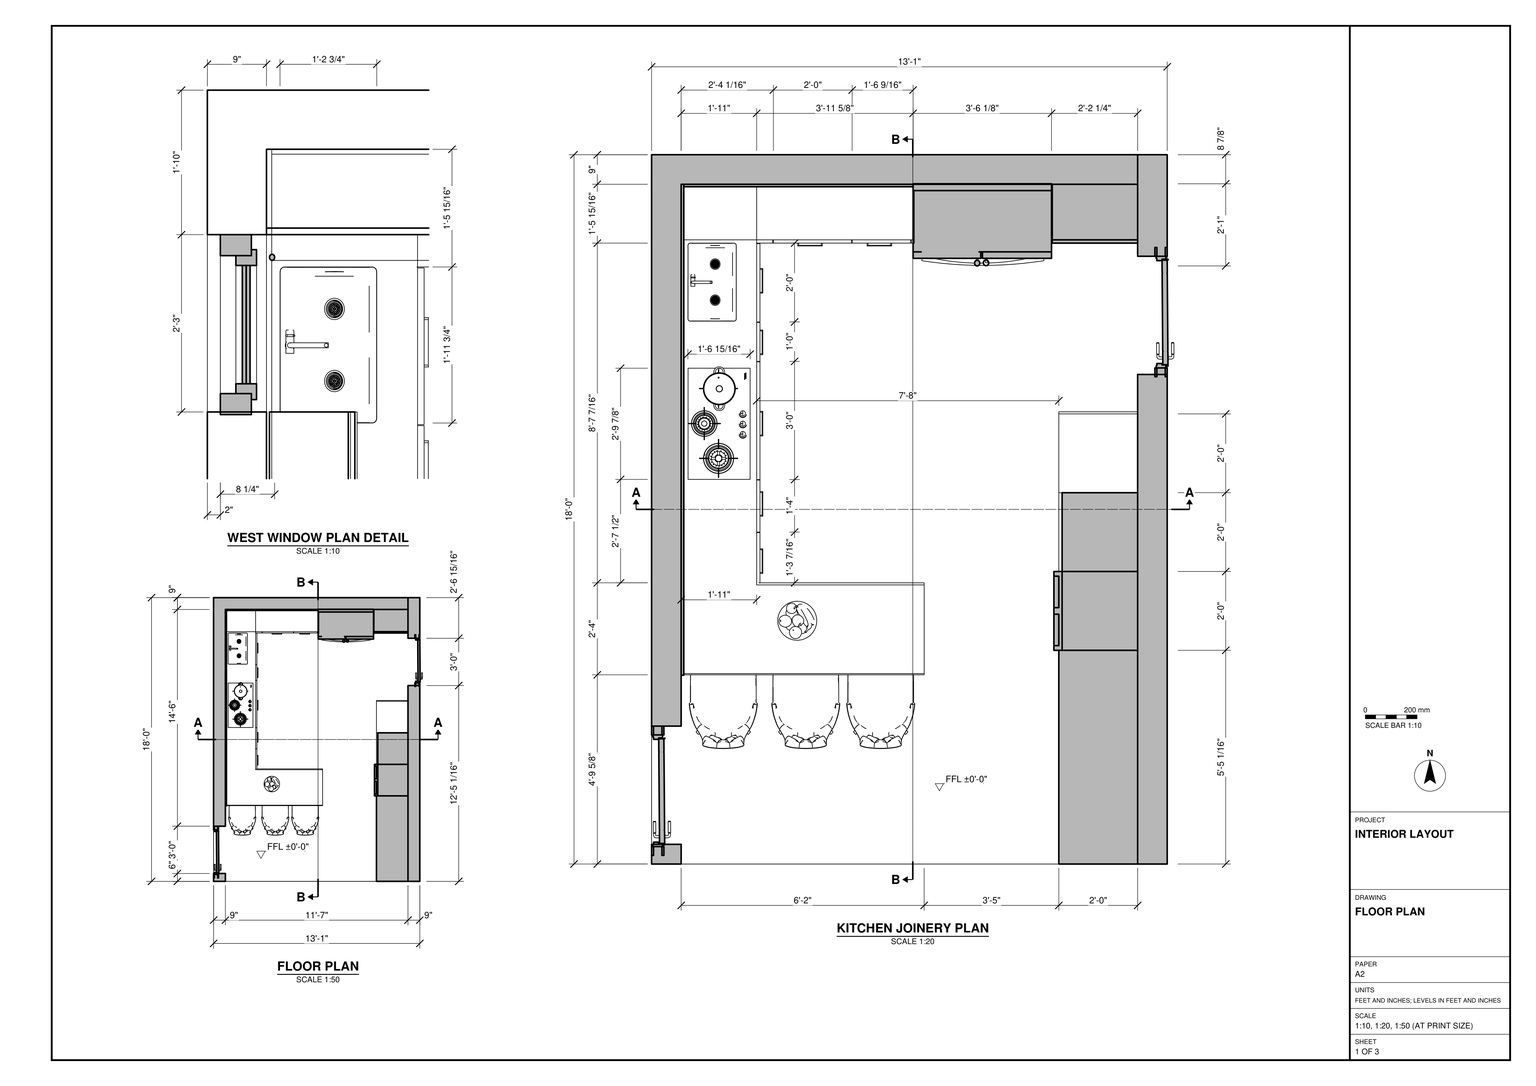
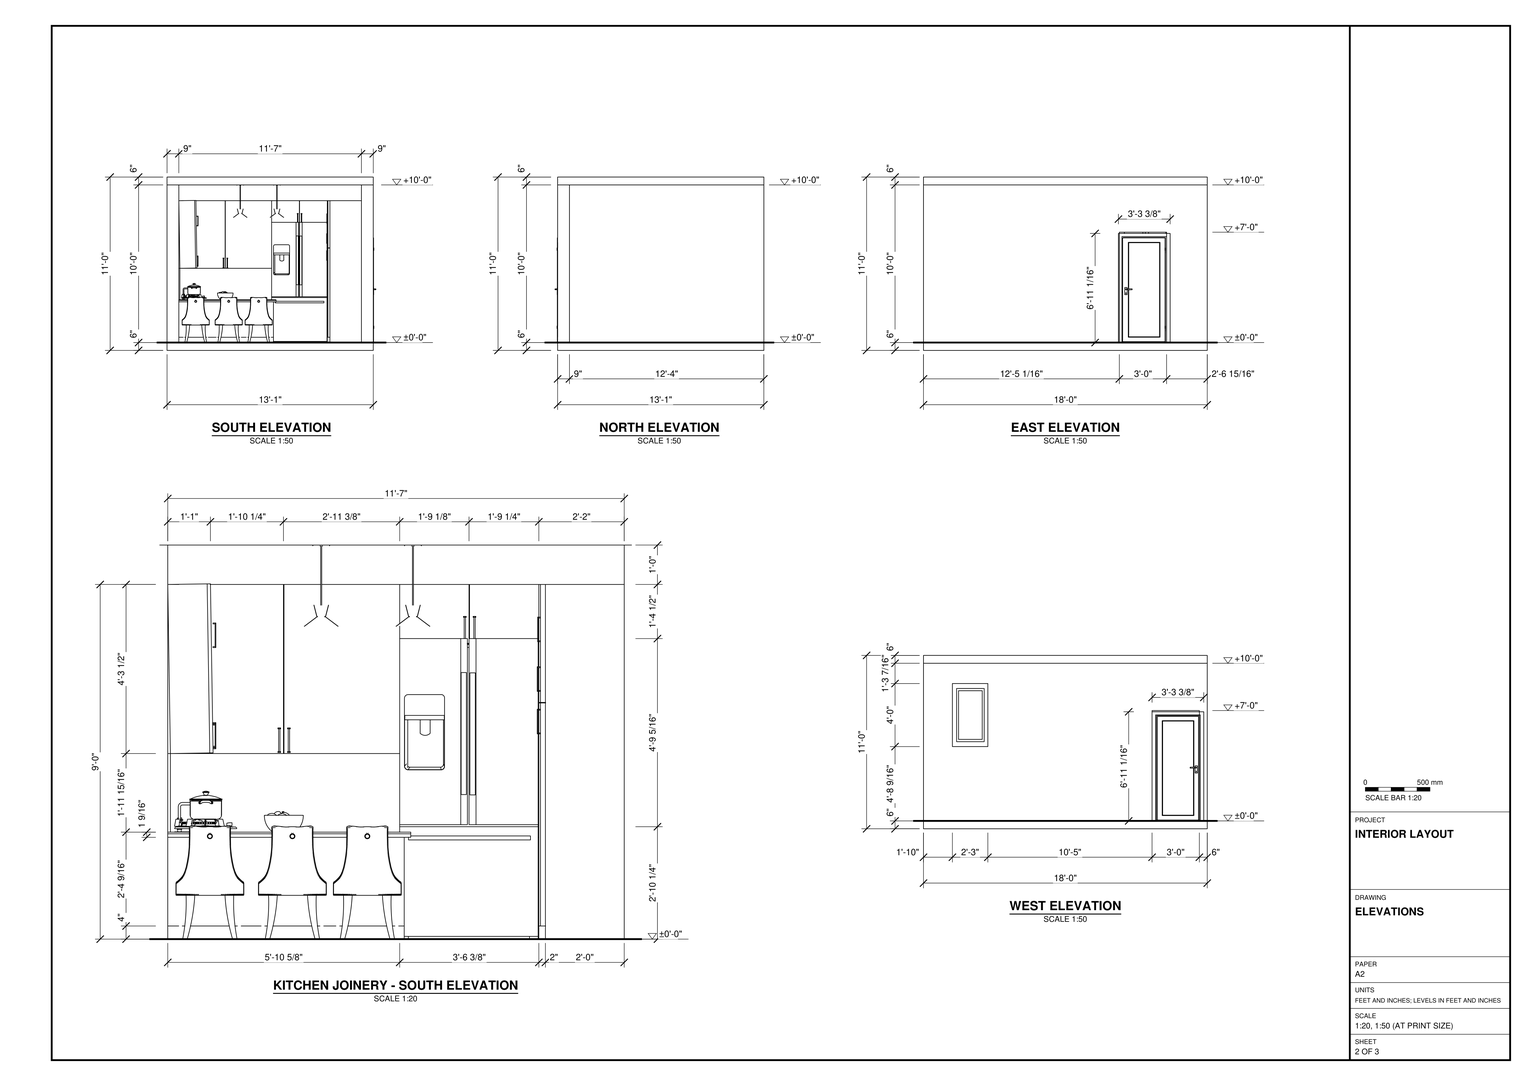
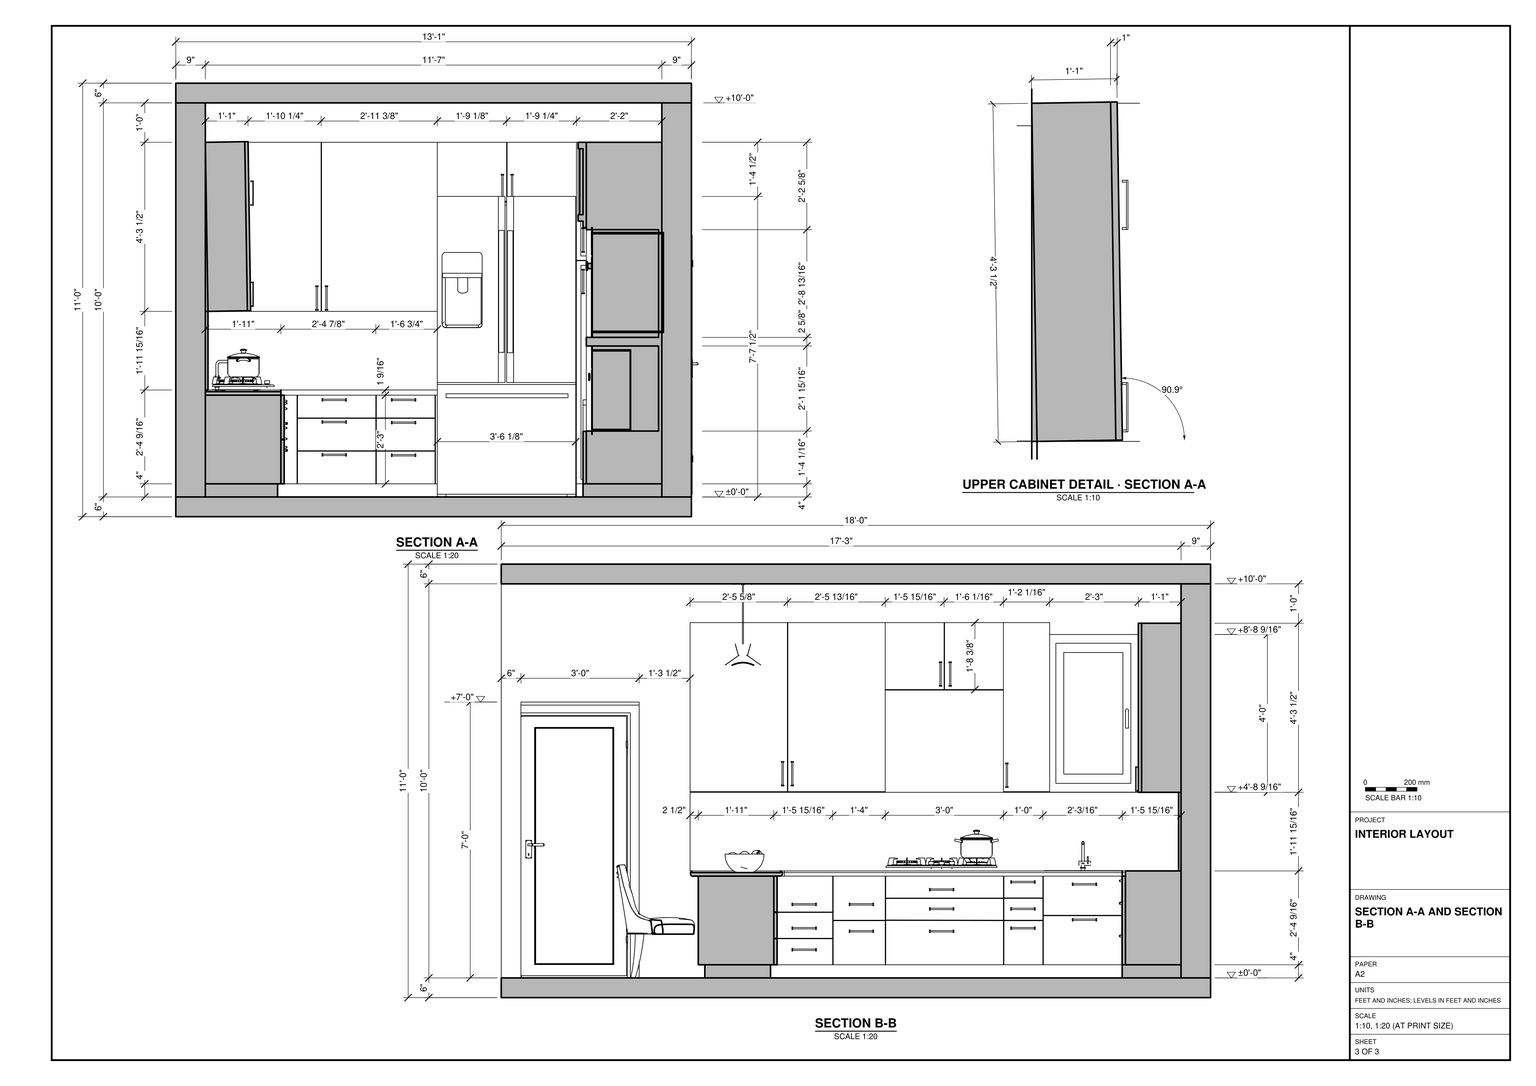
Build the kitchen in SketchUp from task_files/diagram_01.pdf. Work in feet and inches. The overall model extents are 13'-3 1/16" east to west, 18'-0" north to south and 11'-0" high. Set the finished floor of the single storey at ±0'-0". Model the floor slab, roof slab and 9" walls, leaving the south side open as shown. Fit the doors in the east and west walls and use the enlarged plan detail for the west window frame.

Follow the joinery plan for the counter that turns the northwest corner. Place the sink below the window, the cooktop farther south on the west counter and the refrigerator along the north wall. Use the sections to lay out the base unit drawers, cupboard doors, recessed plinths and upper cabinets. Model the tall storage and appliance bays against the east wall. Extend the peninsula from the west run, with three seats along its south edge and a clear passage at its east end.

Keep the shell elements and each furniture or joinery piece in separate groups or components, and use components for repeated parts. Decor, appliances and other loose items may be any suitable library components. Save one SketchUp model as output_files/kitchen_with_fitted_cabinetry_and_seating_peninsula.skp.

# SketchUp Ruby script. Lengths in inches.
U = 1.inch
M = Sketchup.active_model
def pt(a) = Geom::Point3d.new(a.map { |v| v * U })
def face(e, loops, mat)
  f = e.add_face(loops[0].map { |a| pt(a) })
  loops[1..].each { |l| e.add_face(l.map { |a| pt(a) }).erase! }
  f.material = f.back_material = mat if mat
  f
end
# faces: each face lists its corners as indices into pts; further lists are holes
def faces(e, pts, list, mat = nil) = list.each { |f| face(e, (f[0].is_a?(Array) ? f : [f]).map { |l| l.map { |i| pts[i] } }, mat) }
# xy, xz, yz: faces in a plane at the given z, y or x. An outline is a flat list of corners, or four numbers for a rectangle; further outlines are holes
def ring(l) = l.size == 4 ? [[l[0], l[1]], [l[2], l[1]], [l[2], l[3]], [l[0], l[3]]] : l.each_slice(2).to_a
def flat(e, list, mat, &to3) = list.each { |f| face(e, (f[0].is_a?(Array) ? f : [f]).map { |l| ring(l).map { |u, v| to3.(u, v) } }, mat) }
def xy(e, z, list, mat = nil) = flat(e, list, mat) { |x, y| [x, y, z] }
def xz(e, y, list, mat = nil) = flat(e, list, mat) { |x, z| [x, y, z] }
def yz(e, x, list, mat = nil) = flat(e, list, mat) { |y, z| [x, y, z] }
def lines(e, pts, list) = list.each { |a, b| e.add_line(pt(pts[a]), pt(pts[b])) }
# prism: a flat outline (further loops are holes) pulled along v
def prism(e, loops, v, mat = nil)
  f = face(e, loops, mat); d = Geom::Vector3d.new(v.map { |x| x * U })
  f.pushpull(f.normal.samedirection?(d) ? d.length : -d.length)
end
def box(e, o, s, mat = nil) = prism(e, [[o, [o[0] + s[0], o[1], o[2]], [o[0] + s[0], o[1] + s[1], o[2]], [o[0], o[1] + s[1], o[2]]]], [0, 0, s[2]], mat)
def at(x, y, z, deg = 0) = Geom::Transformation.translation(pt([x, y, z])) * Geom::Transformation.rotation(ORIGIN, Z_AXIS, deg.degrees)
def axes(o, x, y, z) = Geom::Transformation.new([*x, 0, *y, 0, *z, 0, *pt(o).to_a, 1])
def part(name) = M.definitions.add(name)
# library, detail: a bought-in or finely detailed component or shape, given as its bounding box
def library(name, o, s) = part(name).tap { |d| box(d.entities, o, s) }
def detail(e, o, s) = box(e.add_group.entities, o, s)
def put(e, d, t, mat = nil) = e.add_instance(d, t).tap { |i| i.material = mat if mat }
def group(e, t, mat = nil) = e.add_group.tap { |g| g.transformation = t; g.material = mat if mat }.entities
root = M.entities
M.materials.add("0202 AP 9417 ROSE ESSENCE").color = [63, 71, 76]
M.materials.add("0209 AP 9428 SKY PINK").color = [243, 236, 233]
M.materials.add("0298 AP 719 GYPSY QUEEN").color = [205, 201, 209]
M.materials.add("0313 AP 7204 FIRST RAY").color = [225, 223, 227]
M.materials.add("[Brick Rough Dark]").color = [94, 77, 53]
M.materials.add("[Color_000]").color = [255, 255, 255]
M.materials.add("[Marble Carrara Floor Tile]").color = [204, 208, 219]
M.materials.add("[Wood Floor]").color = [155, 105, 61]
c1 = library("Component",[0,0,0],[39.37,5.84,83.07])
c2 = part("Composant\#42")
xy(c2.entities,0,[[0,3.54,23.62,8.27]],"[Color_000]")
xy(c2.entities,1.97,[[1.97,2.76,21.65,3.54]],"[Color_000]")
xy(c2.entities,2.76,[[2.76,3.54,20.87,5.91],[2.76,5.91,20.87,8.27]],"[Color_000]")
xy(c2.entities,4.05,[[4.05,2.76,19.58,3.74],[4.05,3.74,19.58,4.33],[4.05,4.33,19.58,4.92],[4.05,4.92,19.58,5.91]],"[Color_000]")
xy(c2.entities,14.39,[[2.97,0,3.07,0.01,3.17,0.05,3.25,0.12,3.3125,0.2,3.35,0.29,3.37,0.39,3.35,0.5,3.3125,0.59,3.25,0.67,3.17,0.73,3.07,0.77,2.97,0.79,2.87,0.77,2.78,0.73,2.69,0.67,2.63,0.59,2.59,0.5,2.58,0.39,2.59,0.29,2.63,0.2,2.69,0.12,2.78,0.05,2.87,0.01]],"[Color_000]")
xy(c2.entities,31.39,[[4.05,2.76,19.58,3.74],[4.05,3.74,19.58,4.33],[4.05,4.33,19.58,4.92],[4.05,4.92,19.58,5.91]],"[Color_000]")
xy(c2.entities,32.68,[[2.76,3.54,20.87,5.91],[2.76,5.91,20.87,8.27]],"[Color_000]")
xy(c2.entities,33.46,[[1.97,2.76,21.65,3.54]],"[Color_000]")
xy(c2.entities,35.43,[[0,3.54,23.62,8.27]],"[Color_000]")
xz(c2.entities,2.76,[[[1.97,1.97,21.65,33.46],[4.05,4.05,19.58,31.39],[2.97,17.93,2.87,17.94,2.78,17.98,2.69,18.04,2.63,18.125,2.59,18.22,2.58,18.32,2.59,18.42,2.63,18.52,2.69,18.6,2.78,18.66,2.87,18.7,2.97,18.72,3.07,18.7,3.17,18.66,3.25,18.6,3.3125,18.52,3.35,18.42,3.37,18.32,3.35,18.22,3.3125,18.125,3.25,18.04,3.17,17.98,3.07,17.94]],[2.97,17.93,3.07,17.94,3.17,17.98,3.25,18.04,3.3125,18.125,3.35,18.22,3.37,18.32,3.35,18.42,3.3125,18.52,3.25,18.6,3.17,18.66,3.07,18.7,2.97,18.72,2.87,18.7,2.78,18.66,2.69,18.6,2.63,18.52,2.59,18.42,2.58,18.32,2.59,18.22,2.63,18.125,2.69,18.04,2.78,17.98,2.87,17.94]],"[Color_000]")
xz(c2.entities,3.54,[[[0,0,23.62,35.43],[1.97,1.97,21.65,33.46]],[[1.97,1.97,21.65,33.46],[2.76,2.76,20.87,32.68]]],"[Color_000]")
xz(c2.entities,3.74,[[4.05,4.05,19.58,31.39]])
xz(c2.entities,4.33,[[4.05,4.05,19.58,31.39]])
xz(c2.entities,4.92,[[4.05,4.05,19.58,31.39]])
xz(c2.entities,5.91,[[[2.76,2.76,20.87,32.68],[4.05,4.05,19.58,31.39]]],"[Color_000]")
xz(c2.entities,8.27,[[[0,0,23.62,35.43],[2.76,2.76,20.87,32.68]]],"[Color_000]")
yz(c2.entities,0,[[3.54,0,8.27,35.43]],"[Color_000]")
yz(c2.entities,1.97,[[2.76,1.97,3.54,33.46]],"[Color_000]")
yz(c2.entities,2.76,[[3.54,2.76,5.91,32.68],[5.91,2.76,8.27,32.68]],"[Color_000]")
yz(c2.entities,4.05,[[2.76,4.05,3.74,31.39],[3.74,4.05,4.33,31.39],[4.33,4.05,4.92,31.39],[4.92,4.05,5.91,31.39]],"[Color_000]")
yz(c2.entities,19.58,[[2.76,4.05,3.74,31.39],[3.74,4.05,4.33,31.39],[4.33,4.05,4.92,31.39],[4.92,4.05,5.91,31.39]],"[Color_000]")
yz(c2.entities,20.87,[[3.54,2.76,5.91,32.68],[5.91,2.76,8.27,32.68]],"[Color_000]")
yz(c2.entities,21.65,[[2.76,1.97,3.54,33.46]],"[Color_000]")
yz(c2.entities,23.62,[[3.54,0,8.27,35.43]],"[Color_000]")
p = [[2.78,0.05,18.66],[2.87,0.01,18.7],[2.87,0.01,14.39],[2.78,0.05,14.39],[2.97,0,18.72],[2.97,0,14.39],
  [3.07,0.01,18.7],[3.07,0.01,14.39],[3.17,0.05,18.66],[3.17,0.05,14.39],[2.63,0.2,18.52],[2.69,0.12,18.6],
  [2.69,0.12,14.39],[2.63,0.2,14.39],[3.25,0.12,18.6],[3.25,0.12,14.39],[3.3125,0.2,18.52],[3.3125,0.2,14.39],
  [2.59,0.29,18.42],[2.59,0.29,14.39],[3.35,0.29,18.42],[3.35,0.29,14.39],[2.58,0.39,18.32],[2.58,0.39,14.39],
  [3.37,0.39,18.32],[3.37,0.39,14.39],[2.59,0.5,18.22],[2.59,0.5,14.39],[3.35,0.5,18.22],[3.35,0.5,14.39],
  [2.63,0.59,18.125],[2.63,0.59,14.39],[3.3125,0.59,18.125],[3.3125,0.59,14.39],[2.69,0.67,18.04],[2.69,0.67,14.39],
  [3.25,0.67,18.04],[3.25,0.67,14.39],[2.78,0.73,17.98],[2.78,0.73,14.39],[2.87,0.77,17.94],[2.87,0.77,14.39],
  [3.17,0.73,17.98],[3.07,0.77,17.94],[3.07,0.77,14.39],[3.17,0.73,14.39],[2.97,0.79,17.93],[2.97,0.79,14.39],
  [2.87,2.76,17.94],[2.78,2.76,17.98],[3.17,2.76,17.98],[3.07,2.76,17.94],[2.97,2.76,17.93],[2.69,2.76,18.04],
  [2.63,2.76,18.125],[3.3125,2.76,18.125],[3.25,2.76,18.04],[2.59,2.76,18.22],[3.35,2.76,18.22],[2.58,2.76,18.32],
  [3.37,2.76,18.32],[2.59,2.76,18.42],[3.35,2.76,18.42],[2.63,2.76,18.52],[3.3125,2.76,18.52],[2.69,2.76,18.6],
  [3.25,2.76,18.6],[2.78,2.76,18.66],[3.17,2.76,18.66],[2.87,2.76,18.7],[2.97,2.76,18.72],[3.07,2.76,18.7],
  [2.76,3.54,2.76],[2.76,2.76,2.76]]
faces(c2.entities,p,[[0,1,2,3],[1,4,5,2],[4,6,7,5],[6,8,9,7],[10,11,12,13],[11,0,3,12],[8,14,15,9],[14,16,17,15],
  [18,10,13,19],[16,20,21,17],[22,18,19,23],[20,24,25,21],[26,22,23,27],[24,28,29,25],[30,26,27,31],[28,32,33,29],
  [34,30,31,35],[32,36,37,33],[38,34,35,39],[40,38,39,41],[42,43,44,45],[36,42,45,37],[46,40,41,47],[43,46,47,44],
  [48,49,38,40],[50,51,43,42],[52,48,40,46],[51,52,46,43],[53,54,30,34],[55,56,36,32],[49,53,34,38],[56,50,42,36],
  [54,57,26,30],[58,55,32,28],[57,59,22,26],[60,58,28,24],[59,61,18,22],[62,60,24,20],[61,63,10,18],[64,62,20,16],
  [63,65,11,10],[66,64,16,14],[65,67,0,11],[68,66,14,8],[67,69,1,0],[69,70,4,1],[70,71,6,4],[71,68,8,6]],"[Color_000]")
lines(c2.entities,p,[[72,73]])
c3 = part("POI-E1497-320-1917\#1")
xy(c3.entities,0,[[0,0,0.29,0.83],[7.21,0,7.5,0.83]])
xy(c3.entities,0.64,[[0.29,0.21,7.21,0.62]])
xy(c3.entities,0.875,[[0,0.21,7.5,0.62]])
xz(c3.entities,0.21,[[0,0.64,7.5,0.875]])
xz(c3.entities,0.62,[[0,0.64,7.5,0.875]])
yz(c3.entities,0,[[0,0,0.21,0.64,0.21,0.875,0.62,0.875,0.62,0.64,0.83,0]])
yz(c3.entities,0.29,[[0,0,0.83,0,0.62,0.64,0.21,0.64]])
yz(c3.entities,7.21,[[0,0,0.21,0.64,0.62,0.64,0.83,0]])
yz(c3.entities,7.5,[[0,0,0.83,0,0.62,0.64,0.62,0.875,0.21,0.875,0.21,0.64]])
p = [[0,0.21,0.64],[0,0,0],[0.29,0,0],[0.29,0.21,0.64],[7.21,0.21,0.64],[7.21,0,0],
  [7.5,0,0],[7.5,0.21,0.64],[0,0.83,0],[0,0.62,0.64],[0.29,0.62,0.64],[0.29,0.83,0],
  [7.5,0.83,0],[7.5,0.62,0.64],[7.21,0.62,0.64],[7.21,0.83,0]]
faces(c3.entities,p,[[0,1,2,3],[4,5,6,7],[8,9,10,11],[12,13,14,15]])
c4 = library("double fridge",[0,-4.28,0],[46.86,25.01,91.52])
c5 = library("TEKA GVI 78 2G AI AL 2TR GAS ON GLASS BUILT-IN HOB",[0,0,-0.47],[34.26,18.94,11.88])
c6 = library("Chimney",[0,-0.01,0],[29.73,15.52,29.75])
c7 = library("sink",[0,0,0],[20.24,32.66,22.26])
c8 = library("chair",[-10.58,-10.47,0],[21.16,24.25,35.18])
c9 = library("vm_v2_031",[-4.73,-4.73,0],[9.46,9.46,3.85])
c10 = library("110",[-2.16,-2.17,0],[9.05,9.06,51.18])
c11 = part("Group\#1")
box(c11.entities,[0,0,0],[157,216,6])
c12 = library("Group\#47",[0,0,0],[23.62,23.48,17.72])
yz(root,122.5,[[66.5,11.43,76.08,76.57],[78.08,11.43,87.65,76.57],[66.5,79.43,76.08,112.57],[78.08,79.43,87.65,112.57]],"0202 AP 9417 ROSE ESSENCE")
put(root,c1,at(0,42,6,-90))
put(root,c1,at(153.26,187.76,6,-90))
put(root,c2,axes([10.24,194,62.57],[0,-1.16,0],[-1,0,0],[0,0,1.35467]))
put(root,c3,axes([22.77,85.27,71.9375],[0,0,-1],[0,1,0],[1,0,0]))
put(root,c3,axes([22.77,88.21,71.9375],[0,0,-1],[0,1,0],[1,0,0]))
put(root,c3,axes([22.77,133.36,102.28],[0,0,-1],[0,1,0],[1,0,0]))
put(root,c3,axes([22.77,136.29,102.28],[0,0,-1],[0,1,0],[1,0,0]))
put(root,c3,axes([22.78,153.56,71.47],[0,0,-1],[0,1,0],[1,0,0]))
put(root,c3,axes([42.54,194,70.32],[0,0,-1],[1,0,0],[0,-1,0]))
put(root,c3,axes([45.48,194,70.32],[0,0,-1],[1,0,0],[0,-1,0]))
put(root,c3,axes([99.05,189.08,104.28],[0,0,-1],[1,0,0],[0,-1,0]))
put(root,c3,axes([101.99,189.08,104.28],[0,0,-1],[1,0,0],[0,-1,0]))
put(root,c3,axes([122.5,100.91,104.0625],[0,0,-1],[0,-1,0],[-1,0,0]))
put(root,c3,axes([122.5,102.03,104.0625],[0,0,-1],[0,-1,0],[-1,0,0]))
put(root,c3,axes([122.375,78.1,88.94],[0,0,-1],[0,-1,0],[-1,0,0]))
put(root,c3,axes([122.375,76.97,88.94],[0,0,-1],[0,-1,0],[-1,0,0]))
put(root,c3,axes([122.375,78.1,76],[0,0,-1],[0,-1,0],[-1,0,0]))
put(root,c3,axes([122.375,76.97,76],[0,0,-1],[0,-1,0],[-1,0,0]))
put(root,c3,axes([123.64,188.89,87.97],[0,0,-1],[1,0,0],[0,-1,0]))
put(root,c3,axes([123.64,189.08,75.34],[0,0,-1],[1,0,0],[0,-1,0]))
put(root,c3,axes([33,95.99,28.8],[0,-1,0],[0,0,-1],[1,0,0]))
put(root,c3,axes([33,95.99,21.55],[0,-1,0],[0,0,-1],[1,0,0]))
put(root,c3,axes([33,95.99,14.99],[0,-1,0],[0,0,-1],[1,0,0]))
put(root,c3,axes([33,113.42,28.8],[0,-1,0],[0,0,-1],[1,0,0]))
put(root,c3,axes([33,113.42,20.62],[0,-1,0],[0,0,-1],[1,0,0]))
put(root,c3,axes([33,137.86,20.62],[0,-1,0],[0,0,-1],[1,0,0]))
put(root,c3,axes([33,137.86,27.43],[0,-1,0],[0,0,-1],[1,0,0]))
put(root,c3,axes([33,137.86,33.3],[0,-1,0],[0,0,-1],[1,0,0]))
put(root,c3,axes([33,162.61,35.62],[0,-1,0],[0,0,-1],[1,0,0]))
put(root,c3,axes([33,162.61,27.43],[0,-1,0],[0,0,-1],[1,0,0]))
put(root,c3,axes([33,162.61,21.55],[0,-1,0],[0,0,-1],[1,0,0]))
put(root,c3,axes([33,181.35,34.93],[0,-1,0],[0,0,-1],[1,0,0]))
put(root,c3,axes([33,181.35,24.12],[0,-1,0],[0,0,-1],[1,0,0]))
put(root,c3,axes([51.98,189.08,35.98],[-1,0,0],[0,0,-1],[0,-1,0]))
put(root,c3,axes([51.98,189.08,29.23],[-1,0,0],[0,0,-1],[0,-1,0]))
put(root,c3,axes([51.98,189.08,19.23],[-1,0,0],[0,0,-1],[0,-1,0]))
put(root,c3,axes([73.11,189.08,35.98],[-1,0,0],[0,0,-1],[0,-1,0]))
put(root,c3,axes([73.11,189.08,29.05],[-1,0,0],[0,0,-1],[0,-1,0]))
put(root,c3,axes([73.11,189.08,19.12],[-1,0,0],[0,0,-1],[0,-1,0]))
put(root,c4,axes([79.625,186.42,6],[0.89957,0,0],[0,1,0],[0,0,1]))
put(root,c5,at(30,117.13,39.64,90))
put(root,c6,at(22.79,119.25,64.59,90))
put(root,c7,axes([11.0625,165.32,31.42],[0.7275,0,0],[0,0.7275,0],[0,0,0.7275]))
put(root,c8,axes([21.83,48.625,6],[-0.98,0,0],[0,-0.98,0],[0,0,0.98]))
put(root,c8,axes([46.95,48.625,6],[-0.98,0,0],[0,-0.98,0],[0,0,0.98]))
put(root,c8,axes([69.77,48.625,6],[-0.98,0,0],[0,-0.98,0],[0,0,0.98]))
put(root,c9,axes([44.34,74.09,38.07],[1.7673,0,0],[0,1.7673,0],[0,0,1.7673]))
put(root,c10,axes([80.97,70.74,101.25],[1.14155,0,0],[0,1.2087,0],[0,0,0.48348]))
put(root,c10,axes([53.03,70.74,101.25],[1.14155,0,0],[0,1.2087,0],[0,0,0.48348]))
put(root,c11,at(0,0,0),"[Wood Floor]")
g1 = group(root,at(0,0,6),"0313 AP 7204 FIRST RAY")
xy(g1,0,[[0,0,9,6],[0,42,0,216,148,216,148,207,9,207,9,42]])
xy(g1,56.57,[[0,167,9,194]])
xy(g1,84,[[0,6,9,42]])
xy(g1,104.57,[[0,167,9,194]])
xy(g1,120,[[0,0,9,0,9,207,148,207,148,216,0,216]])
xz(g1,0,[[0,0,9,120]])
xz(g1,6,[[0,0,9,84]])
xz(g1,42,[[0,0,9,84]])
xz(g1,167,[[0,56.57,9,104.57]])
xz(g1,194,[[0,56.57,9,104.57]])
xz(g1,207,[[9,0,148,120]])
xz(g1,216,[[0,0,148,120]])
yz(g1,0,[[[0,0,0,120,216,120,216,0,42,0,42,84,6,84,6,0],[167,56.57,194,104.57]]])
yz(g1,9,[[[0,0,6,0,6,84,42,84,42,0,207,0,207,120,0,120],[167,56.57,194,104.57]]])
yz(g1,148,[[207,0,216,120]])
g2 = group(root,at(9,60,6),"0313 AP 7204 FIRST RAY")
prism(g2,[[[0,129.08,0],[22,129.08,0],[22,22,0],[72,22,0],[72,2,0],[0,2,0]]],[0,0,4])
g3 = group(root,at(9,60,10),"0313 AP 7204 FIRST RAY")
xy(g3,-7.5,[[3.84,105.96,16.72,117.02],[4.47,117.02,16.66,127.67]])
xy(g3,0,[[0,0,0,129.08,23,129.08,23,23,72,23,72,0]])
xy(g3,27,[[[0,0,72,0,72,23,23,23,23,129.08,0,129.08],[3.84,105.96,3.84,117.02,4.47,117.02,4.47,127.67,16.66,127.67,16.66,117.02,16.72,117.02,16.72,105.96]]])
xz(g3,0,[[0,0,72,27]])
xz(g3,23,[[23,0,72,27]])
xz(g3,105.96,[[3.84,-7.5,16.72,27]])
xz(g3,117.02,[[3.84,-7.5,4.47,27],[4.47,-7.5,16.66,27],[16.66,-7.5,16.72,27]])
xz(g3,127.67,[[4.47,-7.5,16.66,27]])
xz(g3,129.08,[[0,0,23,27]])
yz(g3,0,[[0,0,129.08,27]])
yz(g3,3.84,[[105.96,-7.5,117.02,27]])
yz(g3,4.47,[[117.02,-7.5,127.67,27]])
yz(g3,16.66,[[117.02,-7.5,127.67,27]])
yz(g3,16.72,[[105.96,-7.5,117.02,27]])
yz(g3,23,[[23,0,129.08,27]])
yz(g3,72,[[0,0,23,27]])
g4 = group(root,at(32,83,10))
xy(g4,0,[[0,0,1,17.92],[0,18.08,1,33.92],[0,34.08,1,69.92],[0,70.08,1,81.92],[0,82.08,1,105.92]])
xy(g4,13.42,[[0,18.08,1,33.92],[0,70.08,1,81.92]])
xy(g4,13.58,[[0,18.08,1,33.92],[0,70.08,1,81.92]])
xy(g4,14.92,[[0,82.08,1,105.92]])
xy(g4,15.08,[[0,82.08,1,105.92]])
xy(g4,20.17,[[0,34.08,1,69.92]])
xy(g4,20.21,[[0,70.08,1,81.92]])
xy(g4,20.33,[[0,34.08,1,69.92]])
xy(g4,20.37,[[0,70.08,1,81.92]])
xy(g4,27,[[0,0,1,17.92],[0,18.08,1,33.92],[0,34.08,1,69.92],[0,70.08,1,81.92],[0,82.08,1,105.92]])
xz(g4,0,[[0,0,1,27]])
xz(g4,17.92,[[0,0,1,27]])
xz(g4,18.08,[[0,0,1,13.42],[0,13.58,1,27]])
xz(g4,33.92,[[0,0,1,13.42],[0,13.58,1,27]])
xz(g4,34.08,[[0,0,1,13.5],[0,13.66,1,20.17],[0,20.33,1,27]])
xz(g4,69.92,[[0,0,1,13.42],[0,13.58,1,20.17],[0,20.33,1,27]])
xz(g4,70.08,[[0,0,1,13.42],[0,13.58,1,20.21],[0,20.37,1,27]])
xz(g4,81.92,[[0,0,1,13.42],[0,13.58,1,20.21],[0,20.37,1,27]])
xz(g4,82.08,[[0,0,1,14.92],[0,15.08,1,27]])
xz(g4,105.92,[[0,0,1,14.92],[0,15.08,1,27]])
yz(g4,0,[[0,0,17.92,27],[17.92,0,18.08,27],[18.08,0,33.92,13.42],[33.92,0,34.08,27],[34.08,0,34.08,13.5,69.92,13.42,69.92,0],
  [69.92,0,70.08,27],[70.08,0,81.92,13.42],[81.92,0,82.08,27],[82.08,0,105.92,14.92],[105.92,0,106.08,27],
  [18.08,13.42,33.92,13.58],[69.92,13.42,69.92,13.58,34.08,13.66,34.08,13.5],[70.08,13.42,81.92,13.58],[18.08,13.58,33.92,27],[69.92,13.58,34.08,13.66,34.08,20.17,69.92,20.17],
  [70.08,13.58,81.92,20.21],[82.08,14.92,105.92,15.08],[82.08,15.08,105.92,27],[34.08,20.17,69.92,20.33],[70.08,20.21,81.92,20.37],
  [34.08,20.33,69.92,27],[70.08,20.37,81.92,27]])
yz(g4,1,[[0,0,17.92,27],[18.08,0,33.92,13.42],[34.08,0,69.92,0,69.92,13.42,34.08,13.5],[70.08,0,81.92,13.42],[82.08,0,105.92,14.92],
  [18.08,13.58,33.92,27],[69.92,13.58,69.92,20.17,34.08,20.17,34.08,13.66],[70.08,13.58,81.92,20.21],[82.08,15.08,105.92,27],[34.08,20.33,69.92,27],
  [70.08,20.37,81.92,27]])
p = [[1,34.08,13.5],[1,69.92,13.42],[0,69.92,13.42],[0,34.08,13.5],[1,69.92,13.58],[1,34.08,13.66],
  [0,34.08,13.66],[0,69.92,13.58],[1,17.92,8.08],[1,1,8.08],[1,17.92,16.08],[1,1,16.08],
  [1,17.92,7.92],[1,1,7.92],[1,17.92,15.92],[1,1,15.92],[1,70.08,13.5],[1,69.92,13.5],
  [1,34.08,13.58],[1,33.92,13.58]]
faces(g4,p,[[0,1,2,3],[4,5,6,7]])
lines(g4,p,[[8,9],[10,11],[12,13],[14,15],[16,17],[18,19]])
g5 = group(root,at(32,83,10))
xy(g5,0,[[0,0,24.92,1],[25.08,0,49,1]])
xy(g5,7.92,[[25.08,0,49,1]])
xy(g5,8.08,[[25.08,0,49,1]])
xy(g5,15.92,[[25.08,0,49,1]])
xy(g5,16.08,[[25.08,0,49,1]])
xy(g5,27,[[0,0,24.92,1],[25.08,0,49,1]])
xz(g5,0,[[0,0,24.92,27],[24.92,0,25.08,27],[25.08,0,49,7.92],[25.08,7.92,49,8.08],[25.08,8.08,49,15.92],
  [25.08,15.92,49,16.08],[25.08,16.08,49,27]])
xz(g5,1,[[0,0,24.92,27],[25.08,0,49,7.92],[25.08,8.08,49,15.92],[25.08,16.08,49,27]])
yz(g5,0,[[0,0,1,27]])
yz(g5,24.92,[[0,0,1,27]])
yz(g5,25.08,[[0,0,1,7.92],[0,8.08,1,15.92],[0,16.08,1,27]])
yz(g5,49,[[0,0,1,7.92],[0,8.08,1,15.92],[0,16.08,1,27]])
p = [[24.92,1,8],[25.08,1,8],[1,1,8],[24.92,1,16],[0.98,1,16]]
lines(g5,p,[[0,1],[0,2],[3,4]])
g6 = group(root,at(9,57.5,38.57),"[Marble Carrara Floor Tile]")
box(g6,[0,0,0],[0.8,149.5,23.9375])
g7 = group(root,at(9,189.08,10),"0298 AP 719 GYPSY QUEEN")
box(g7,[0,1,0],[70.625,16.92,28.57])
g8 = group(root,at(9,189.08,37))
xz(g8,0,[[23,0,70.625,1.57]])
yz(g8,23,[[0,0,17.92,1.57]])
yz(g8,70.625,[[0,0,16,1.57]])
yz(g8,113,[[16,0,17.92,1.57]])
p = [[113,17.92,0],[23,17.92,0]]
lines(g8,p,[[0,1]])
g9 = group(root,at(9,60,37),"0298 AP 719 GYPSY QUEEN")
xy(g9,0,[[[0,-2,0,147,23,147,23,25,74,25,74,-2],[3.53,106.29,15.64,128.4]]])
xy(g9,1.07,[[[0,-2,74,-2,74,25,23,25,23,147,0,147],[3.53,106.29,15.64,128.4]]])
xz(g9,-2,[[0,1.07,74,1.57]])
xz(g9,25,[[23,1.07,74,1.57]])
xz(g9,106.29,[[3.53,0,15.64,1.07]])
xz(g9,128.4,[[3.53,0,15.64,1.07]])
xz(g9,147,[[0,0,23,1.07]])
yz(g9,0,[[-2,0,-2.11,0.1,-2.2,0.22,-2.28,0.35,-2.33,0.49,-2.36,0.64,-2.375,0.79,-2.36,0.9375,-2.33,1.08,-2.28,1.22,-2.2,1.35,-2.11,1.47,-2,1.57],[-2,0,147,1.07]])
yz(g9,3.53,[[106.29,0,128.4,1.07]])
yz(g9,15.64,[[106.29,0,128.4,1.07]])
yz(g9,23,[[25,1.07,147,1.57]])
yz(g9,74,[[-2,0,25,0,25.17,0.06,25.32,0.16,25.45,0.28,25.55,0.4375,25.6,0.61,25.625,0.79,25.6,0.97,25.55,1.14,25.45,1.29,25.32,1.42,25.17,1.51,25,1.57,25,1.07,-2,1.07,-2,1.57,-2.11,1.47,-2.2,1.35,-2.28,1.22,-2.33,1.08,-2.36,0.9375,-2.375,0.79,-2.36,0.64,-2.33,0.49,-2.28,0.35,-2.2,0.22,-2.11,0.1]])
p = [[74,-2,0],[74,-2.11,0.1],[0,-2.11,0.1],[0,-2,0],[74,25.17,0.06],[74,25,0],
  [23,25,0],[23.17,25.17,0.06],[74,-2.2,0.22],[0,-2.2,0.22],[74,25.32,0.16],[23.32,25.32,0.16],
  [74,-2.28,0.35],[0,-2.28,0.35],[74,25.45,0.28],[23.45,25.45,0.28],[74,25.55,0.4375],[23.55,25.55,0.4375],
  [74,-2.33,0.49],[0,-2.33,0.49],[74,25.6,0.61],[23.6,25.6,0.61],[74,-2.36,0.64],[0,-2.36,0.64],
  [74,-2.375,0.79],[0,-2.375,0.79],[74,25.625,0.79],[23.625,25.625,0.79],[74,-2.36,0.9375],[0,-2.36,0.9375],
  [74,25.6,0.97],[23.6,25.6,0.97],[74,-2.33,1.08],[0,-2.33,1.08],[74,25.55,1.14],[23.55,25.55,1.14],
  [74,-2.28,1.22],[0,-2.28,1.22],[74,25.45,1.29],[23.45,25.45,1.29],[74,-2.2,1.35],[0,-2.2,1.35],
  [74,25.32,1.42],[23.32,25.32,1.42],[74,-2.11,1.47],[0,-2.11,1.47],[74,25.17,1.51],[23.17,25.17,1.51],
  [74,-2,1.57],[0,-2,1.57],[74,25,1.57],[23,25,1.57]]
faces(g9,p,[[0,1,2,3],[4,5,6,7],[1,8,9,2],[10,4,7,11],[8,12,13,9],[14,10,11,15],[16,14,15,17],[12,18,19,13],
  [20,16,17,21],[18,22,23,19],[22,24,25,23],[26,20,21,27],[24,28,29,25],[30,26,27,31],[28,32,33,29],[34,30,31,35],
  [32,36,37,33],[38,34,35,39],[36,40,41,37],[42,38,39,43],[40,44,45,41],[46,42,43,47],[44,48,49,45],[50,46,47,51]])
g10 = group(root,at(9,189.08,6),"0313 AP 7204 FIRST RAY")
box(g10,[0,0,0],[70.625,17.92,4])
box(g10,[113,0,0],[26,17.92,4])
p = [[113,17.92,0],[70.625,17.92,0]]
lines(g10,p,[[0,1]])
g11 = group(root,at(9,189.08,10))
xy(g11,0,[[0,0,27.9,1],[28.08,0,51.9,1],[52.07,0,69.92,1],[70.08,0,70.625,1]])
xy(g11,9.92,[[28.08,0,51.9,1],[52.07,0,69.92,1]])
xy(g11,10.08,[[28.08,0,51.9,1],[52.07,0,69.92,1]])
xy(g11,19.92,[[28.08,0,51.9,1],[52.07,0,69.92,1]])
xy(g11,20.08,[[28.08,0,51.9,1],[52.07,0,69.92,1]])
xy(g11,27,[[0,0,27.9,1],[28.08,0,51.9,1],[52.07,0,69.92,1],[70.08,0,70.625,1]])
xz(g11,0,[[0,0,27.9,27],[28.08,0,51.9,9.92],[52.07,0,69.92,9.92],[70.08,0,70.625,27],[28.08,10.08,51.9,19.92],
  [52.07,10.08,69.92,19.92],[28.08,20.08,51.9,27],[52.07,20.08,69.92,27]])
xz(g11,1,[[0,0,27.9,27],[27.9,0,28.08,27],[28.08,0,51.9,9.92],[51.9,0,52.07,27],[52.07,0,69.92,9.92],
  [69.92,0,70.08,27],[70.08,0,70.625,27],[28.08,9.92,51.9,10.08],[52.07,9.92,69.92,10.08],[28.08,10.08,51.9,19.92],
  [52.07,10.08,69.92,19.92],[28.08,19.92,51.9,20.08],[52.07,19.92,69.92,20.08],[28.08,20.08,51.9,27],[52.07,20.08,69.92,27]])
yz(g11,0,[[0,0,1,27]])
yz(g11,27.9,[[0,0,1,27]])
yz(g11,28.08,[[0,0,1,9.92],[0,10.08,1,19.92],[0,20.08,1,27]])
yz(g11,51.9,[[0,0,1,9.92],[0,10.08,1,19.92],[0,20.08,1,27]])
yz(g11,52.07,[[0,0,1,9.92],[0,10.08,1,19.92],[0,20.08,1,27]])
yz(g11,69.92,[[0,0,1,9.92],[0,10.08,1,19.92],[0,20.08,1,27]])
yz(g11,70.08,[[0,0,1,27]])
yz(g11,70.625,[[0,0,1,27]])
g12 = group(root,at(79.625,189.08,10),"0209 AP 9428 SKY PINK")
xy(g12,85.7,[[0.22,1,42.15,16]])
xy(g12,104,[[0,1,42.375,17.92]])
xz(g12,16,[[0.22,0.22,42.15,85.7]])
xz(g12,17.92,[[0,0,42.375,104]])
yz(g12,0,[[1,0,17.92,104]])
yz(g12,0.22,[[1,0.22,16,85.7]])
yz(g12,42.15,[[1,0.22,16,85.7]])
yz(g12,42.375,[[1,0,17.92,104]])
g13 = group(root,at(122,189.08,10),"0209 AP 9428 SKY PINK")
box(g13,[0,1,0],[26,16.92,104])
g14 = group(root,at(79.625,189.08,10),"0209 AP 9428 SKY PINK")
xy(g14,0.22,[[0,0,0.22,1]])
xy(g14,85.7,[[0,0,0.22,1],[0.22,0,42.15,1]])
xy(g14,85.92,[[0,0,42.375,1]])
xy(g14,86.08,[[0,0,21.11,1],[21.27,0,42.375,1]])
xy(g14,104,[[0,0,21.11,1],[21.27,0,42.375,1]])
xz(g14,0,[[0,0.22,0.22,85.7],[0,86.08,21.11,104],[21.27,86.08,42.375,104]])
xz(g14,1,[[0,0.22,0.22,85.7],[0,85.92,42.375,86.08],[0,86.08,21.11,104],[21.11,86.08,21.27,104],[21.27,86.08,42.375,104]])
yz(g14,0,[[0,0,1,0.22],[0,0.22,1,85.7],[0,85.7,1,85.92],[0,86.08,1,104]])
yz(g14,0.22,[[0,0.22,1,85.7]])
yz(g14,21.11,[[0,86.08,1,104]])
yz(g14,21.27,[[0,86.08,1,104]])
yz(g14,42.15,[[0,0.22,1,85.7]])
yz(g14,42.375,[[0,0,1,85.92],[0,86.08,1,104]])
g15 = group(root,at(122,189.08,10),"0209 AP 9428 SKY PINK")
xy(g15,0,[[0,0,26,1]])
xy(g15,67.92,[[0,0,26,1]])
xy(g15,68.08,[[0,0,24,1]])
xy(g15,104,[[0,0,24,1]])
xz(g15,0,[[[0,0,26,67.92],[1.38,1.38,24.62,66.54]],[1.38,1.38,24.62,66.54],[[0,68.08,24,104],[1.32,69.4,22.68,102.68]],[1.32,69.4,22.68,102.68]])
xz(g15,1,[[0,0,26,67.92],[0,67.92,24,68.08],[0,68.08,24,104]])
yz(g15,0,[[0,0,1,67.92],[0,68.08,1,104]])
yz(g15,24,[[0,68.08,1,104]])
yz(g15,26,[[0,0,1,67.92]])
g16 = group(root,at(148,0,6),"0313 AP 7204 FIRST RAY")
prism(g16,[[[9,185.08,0],[9,216,0],[9,216,120],[9,0,120],[9,0,0],[9,149.08,0],[9,149.08,84],[9,185.08,84]]],[-9,0,0])
g17 = group(root,at(124,65.08,6))
prism(g17,[[[0,72,0],[0,0,0],[0,0,4],[0,24,4],[0,48,4],[0,72,4]]],[24,0,0])
g18 = group(root,at(124,113.08,10),"0202 AP 9417 ROSE ESSENCE")
box(g18,[1,0,0],[23,24,24])
g19 = group(root,at(124,113.08,34))
xy(g19,0,[[0,0,24,24]])
xy(g19,1.57,[[0,0,24,24]])
xz(g19,0,[[0,0,24,1.57]])
yz(g19,0,[[0,0,0,1.57,24,1.57,24.17,1.51,24.32,1.42,24.45,1.29,24.55,1.14,24.6,0.97,24.625,0.79,24.6,0.61,24.55,0.4375,24.45,0.28,24.32,0.16,24.17,0.06,24,0]])
yz(g19,24,[[0,0,24,1.57],[24,0,24.17,0.06,24.32,0.16,24.45,0.28,24.55,0.4375,24.6,0.61,24.625,0.79,24.6,0.97,24.55,1.14,24.45,1.29,24.32,1.42,24.17,1.51,24,1.57]])
p = [[0,24,0],[0,24.17,0.06],[24,24.17,0.06],[24,24,0],[0,24.32,0.16],[24,24.32,0.16],
  [0,24.45,0.28],[24,24.45,0.28],[0,24.55,0.4375],[24,24.55,0.4375],[0,24.6,0.61],[24,24.6,0.61],
  [0,24.625,0.79],[24,24.625,0.79],[0,24.6,0.97],[24,24.6,0.97],[0,24.55,1.14],[24,24.55,1.14],
  [0,24.45,1.29],[24,24.45,1.29],[0,24.32,1.42],[24,24.32,1.42],[0,24.17,1.51],[24,24.17,1.51],
  [0,24,1.57],[24,24,1.57]]
faces(g19,p,[[0,1,2,3],[1,4,5,2],[4,6,7,5],[6,8,9,7],[8,10,11,9],[10,12,13,11],[12,14,15,13],[14,16,17,15],
  [16,18,19,17],[18,20,21,19],[20,22,23,21],[22,24,25,23]])
g20 = group(root,at(124,89.08,10),"0202 AP 9417 ROSE ESSENCE")
xy(g20,0,[[1,0,24,24]])
xy(g20,16.07,[[1,0.9,23,23.4]])
xy(g20,41.98,[[1,0.9,23,23.4]])
xy(g20,44.6,[[1,0.6,23,23.4]])
xy(g20,77.4,[[1,0.6,23,23.4]])
xy(g20,104,[[1,0,24,24]])
xz(g20,0,[[1,0,24,104]])
xz(g20,0.6,[[1,44.6,23,77.4]])
xz(g20,0.9,[[1,16.07,23,41.98]])
xz(g20,23.4,[[1,16.07,23,41.98],[1,44.6,23,77.4]])
xz(g20,24,[[1,0,24,104]])
yz(g20,1,[[0,0,24,15.23],[[0,15.23,24,44],[0.9,16.07,23.4,41.98]],[[0,44,24,78],[0.6,44.6,23.4,77.4]],[0,78,24,104]])
yz(g20,23,[[0.9,16.07,23.4,41.98],[0.6,44.6,23.4,77.4]])
yz(g20,24,[[0,0,24,104]])
g21 = group(root,at(124,65.08,10),"0202 AP 9417 ROSE ESSENCE")
box(g21,[1,0,0],[23,24,104])
g22 = group(root,at(124,89.08,10),"0202 AP 9417 ROSE ESSENCE")
box(g22,[0,0,0],[1,24,15.98])
xy(g22,78,[[0,0,1,24]])
xy(g22,80,[[-1.5,0,0,24]])
xy(g22,81.96,[[-1.5,1.96,-1,11],[-1,1.96,0,11],[-1.5,13,-1,22.04],[-1,13,0,22.04]])
xy(g22,102.04,[[-1.5,1.96,-1,11],[-1,1.96,0,11],[-1.5,13,-1,22.04],[-1,13,0,22.04]])
xy(g22,104,[[-1.5,0,1,24]])
xz(g22,0,[[0,78,1,78,1,104,-1.5,104,-1.5,80,0,80]])
xz(g22,1.96,[[-1.5,81.96,-1,102.04],[-1,81.96,0,102.04]])
xz(g22,11,[[-1.5,81.96,-1,102.04],[-1,81.96,0,102.04]])
xz(g22,13,[[-1.5,81.96,-1,102.04],[-1,81.96,0,102.04]])
xz(g22,22.04,[[-1.5,81.96,-1,102.04],[-1,81.96,0,102.04]])
xz(g22,24,[[0,78,0,80,-1.5,80,-1.5,104,1,104,1,78]])
yz(g22,-1.5,[[[0,80,24,104],[1.96,81.96,22.04,102.04]],[11,81.96,13,102.04]])
yz(g22,-1,[[1.96,81.96,11,102.04],[13,81.96,22.04,102.04]])
yz(g22,0,[[0,78,24,80],[1.96,81.96,11,102.04],[13,81.96,22.04,102.04]])
yz(g22,1,[[0,78,24,104]])
p = [[1,24,44],[1,24,78],[1,0,44],[1,0,78]]
lines(g22,p,[[0,1],[2,3]])
g23 = group(root,at(124,65.08,10),"0202 AP 9417 ROSE ESSENCE")
xy(g23,0,[[-1.5,0,1,24]])
xy(g23,1.43,[[-1.5,1.43,0,11],[-1.5,13,0,22.57]])
xy(g23,66.57,[[-1.5,1.43,0,11],[-1.5,13,0,22.57]])
xy(g23,67.92,[[-1.5,0,1,24]])
xy(g23,68.08,[[-1.5,0,1,24]])
xy(g23,69.43,[[-1.5,1.43,0,11],[-1.5,13,0,22.57]])
xy(g23,102.57,[[-1.5,1.43,0,11],[-1.5,13,0,22.57]])
xy(g23,104,[[-1.5,0,1,24]])
xz(g23,0,[[-1.5,0,1,67.92],[-1.5,68.08,1,104]])
xz(g23,1.43,[[-1.5,1.43,0,66.57],[-1.5,69.43,0,102.57]])
xz(g23,11,[[-1.5,1.43,0,66.57],[-1.5,69.43,0,102.57]])
xz(g23,13,[[-1.5,1.43,0,66.57],[-1.5,69.43,0,102.57]])
xz(g23,22.57,[[-1.5,1.43,0,66.57],[-1.5,69.43,0,102.57]])
xz(g23,24,[[-1.5,0,1,67.92],[-1.5,68.08,1,104]])
yz(g23,-1.5,[[[0,0,24,67.92],[1.43,1.43,22.57,66.57]],[11,1.43,13,66.57],[[0,68.08,24,104],[1.43,69.43,22.57,102.57]],[11,69.43,13,102.57]])
yz(g23,0,[[1.43,1.43,11,66.57],[13,1.43,22.57,66.57],[1.43,69.43,11,102.57],[13,69.43,22.57,102.57]])
yz(g23,1,[[0,0,24,67.92],[0,67.92,24,68.08],[0,68.08,24,104]])
g24 = group(root,at(124,0,6),"[Brick Rough Dark]")
xy(g24,0,[[0,0,24,65.08]])
xy(g24,108,[[0,0,24,65.08]],"0202 AP 9417 ROSE ESSENCE")
xz(g24,0,[[0,0,24,108]])
xz(g24,65.08,[[0,0,24,108]])
yz(g24,0,[[0,0,65.08,108]])
yz(g24,24,[[0,0,65.08,108]])
g25 = group(root,at(9.8,85,37),"[Marble Carrara Floor Tile]")
xy(g25,1.57,[[0,121.25,22.2,122],[22.2,121.25,69.82,122]])
xy(g25,25.51,[[0,121.25,69.82,122]])
xz(g25,121.25,[[0,1.57,69.82,25.51]])
xz(g25,122,[[0,1.57,69.82,25.51]])
yz(g25,0,[[121.25,1.57,122,25.51]])
yz(g25,22.2,[[1.22,0,104.08,1.57],[104.08,0,122,1.57]])
yz(g25,69.82,[[121.25,1.57,122,25.51]])
p = [[22.2,0,1.57],[22.2,1.22,1.57],[22.2,1.22,0],[22.2,0.39,0]]
lines(g25,p,[[0,1],[2,3]])
g26 = group(root,at(9,195,62.51),"0209 AP 9428 SKY PINK")
box(g26,[0,0,0],[70.625,12,51.49])
g27 = group(root,at(9,194,62.51),"0209 AP 9428 SKY PINK")
xy(g27,0,[[0,0,35.23,1],[35.39,0,70.625,1]])
xy(g27,51.49,[[0,0,35.23,1],[35.39,0,70.625,1]])
xz(g27,0,[[0,0,35.23,51.49],[35.39,0,70.625,51.49]])
xz(g27,1,[[0,0,35.23,51.49],[35.23,0,35.39,51.49],[35.39,0,70.625,51.49]])
yz(g27,0,[[0,0,1,51.49]])
yz(g27,35.23,[[0,0,1,51.49]])
yz(g27,35.39,[[0,0,1,51.49]])
yz(g27,70.625,[[0,0,1,51.49]])
g28 = group(root,at(9,57.5,62.51),"0209 AP 9428 SKY PINK")
xz(g28,0,[[0.8,0,12.8,0.1875,12,51.67,0,51.49]])
xz(g28,59.42,[[1.8,0.02,1.32,31.12,12.32,31.29,12.8,0.1875]])
xz(g28,95.42,[[1.8,0.02,12.8,0.1875,12.32,31.29,1.32,31.12]])
xz(g28,109.5,[[0.8,0,0,51.49,12,51.67,12.8,0.1875]])
p = [[0.8,109.5,0],[0.8,0,0],[0,0,51.49],[0,109.5,51.49],[12.8,109.5,0.1875],[12.8,95.42,0.1875],
  [1.8,95.42,0.02],[1.8,59.42,0.02],[12.8,59.42,0.1875],[12.8,0,0.1875],[1.32,95.42,31.12],[1.32,59.42,31.12],
  [12.32,59.42,31.29],[12,59.42,51.67],[12,0,51.67],[12,109.5,51.67],[12,95.42,51.67],[12.32,95.42,31.29]]
faces(g28,p,[[0,1,2,3],[1,0,4,5,6,7,8,9],[6,10,11,7],[9,8,12,13,14],[15,16,17,5,4],[17,12,11,10],[13,12,17,16],[3,2,14,13,16,15]])
g29 = group(root,at(21,57.5,62.7),"0209 AP 9428 SKY PINK")
xz(g29,0,[[0.8,0,1.8,0.02,1,51.5,0,51.49]])
xz(g29,29.63,[[0.8,0,0,51.49,1,51.5,1.8,0.02]])
xz(g29,29.79,[[0.8,0,1.8,0.02,1,51.5,0,51.49]])
xz(g29,59.42,[[0.8,0,0,51.49,1,51.5,1.8,0.02]])
p = [[0,0,51.49],[0,29.63,51.49],[0.8,29.63,0],[0.8,0,0],[1.8,29.63,0.02],[1.8,0,0.02],
  [1,29.63,51.5],[1,0,51.5],[0,29.79,51.49],[0.8,29.79,0],[0.8,59.42,0],[0,59.42,51.49],
  [1.8,29.79,0.02],[1.8,59.42,0.02],[1,59.42,51.5],[1,29.79,51.5]]
faces(g29,p,[[0,1,2,3],[3,2,4,5],[5,4,6,7],[8,1,2,9],[10,9,8,11],[12,9,10,13],[14,15,12,13],[6,1,0,7],
  [11,8,15,14]])
g30 = group(root,at(21,152.92,62.7),"0209 AP 9428 SKY PINK")
prism(g30,[[[0.8,0,0],[0.8,14.08,0],[1.8,14.08,0.02],[1.8,0,0.02]]],[-0.8,0,51.49])
g31 = group(root,at(21,116.92,93.8),"0209 AP 9428 SKY PINK")
xz(g31,0,[[0.32,0,1.32,0.02,1,20.4,0,20.38]])
xz(g31,17.92,[[0.32,0,0,20.38,1,20.4,1.32,0.02]])
xz(g31,18.08,[[0.32,0,1.32,0.02,1,20.4,0,20.38]])
xz(g31,36,[[0.32,0,0,20.38,1,20.4,1.32,0.02]])
p = [[0,0,20.38],[0,17.92,20.38],[0.32,17.92,0],[0.32,0,0],[1.32,17.92,0.02],[1.32,0,0.02],
  [1,17.92,20.4],[1,0,20.4],[0,18.08,20.38],[0.32,18.08,0],[0.32,36,0],[0,36,20.38],
  [1.32,18.08,0.02],[1.32,36,0.02],[1,36,20.4],[1,18.08,20.4]]
faces(g31,p,[[0,1,2,3],[3,2,4,5],[5,4,6,7],[8,1,2,9],[10,9,8,11],[12,9,10,13],[14,15,12,13],[6,1,0,7],
  [11,8,15,14]])
g32 = group(root,at(124,113.08,10),"0202 AP 9417 ROSE ESSENCE")
xy(g32,0,[[0,0,1,24]])
xy(g32,7.92,[[0,0,1,24]])
xy(g32,8.08,[[0,0,1,24]])
xy(g32,15.92,[[0,0,1,24]])
xy(g32,16.08,[[0,0,1,24]])
xy(g32,24,[[0,0,1,24]])
xz(g32,0,[[0,0,1,7.92],[0,8.08,1,15.92],[0,16.08,1,24]])
xz(g32,24,[[0,0,1,7.92],[0,8.08,1,15.92],[0,16.08,1,24]])
yz(g32,0,[[0,0,24,7.92],[0,8.08,24,15.92],[0,16.08,24,24]])
yz(g32,1,[[0,0,24,7.92],[0,7.92,24,8.08],[0,8.08,24,15.92],[0,15.92,24,16.08],[0,16.08,24,24]])
put(root,c11,at(0,0,126),"0313 AP 7204 FIRST RAY")
put(root,c12,axes([125,113.3,54.6],[0,-1,0],[1,0,0],[0,0,1.8853]))
put(root,c12,axes([125.8,112.48,25.0625],[0,-0.99065,0],[0.54,0,0],[0,0,1.5191]))
